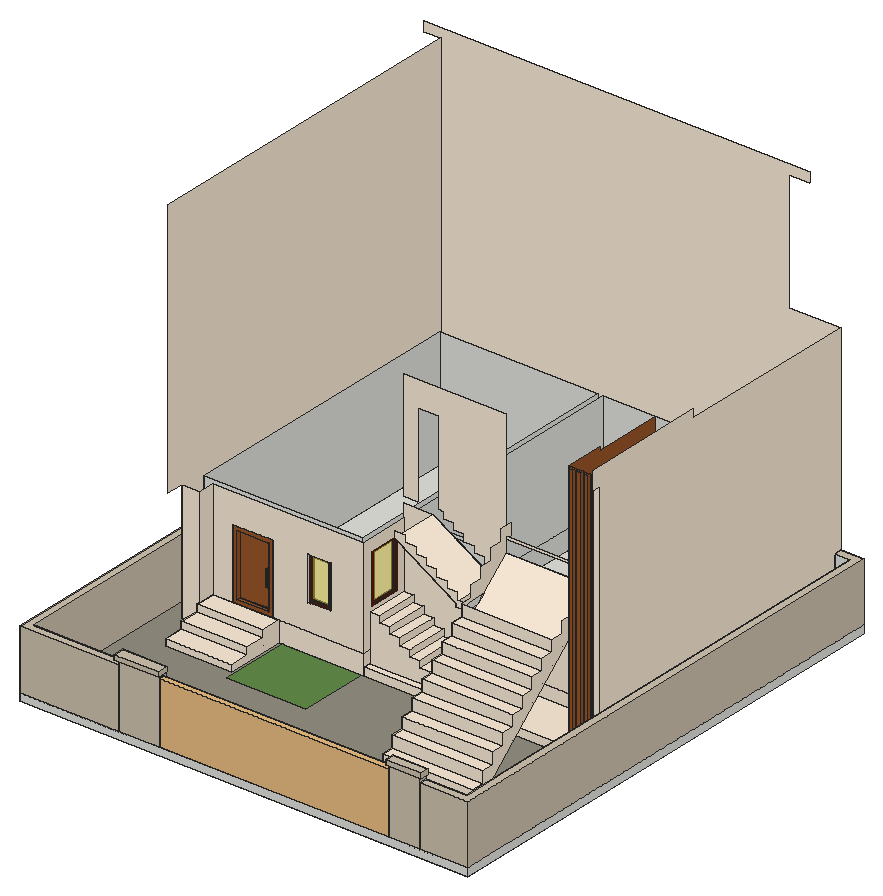
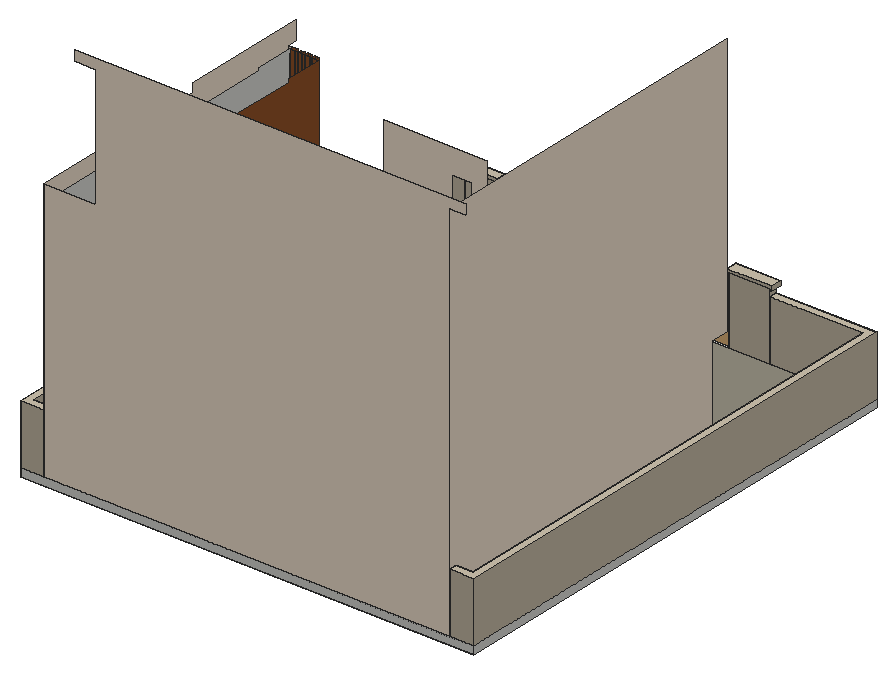
# SketchUp Ruby script. Lengths in inches.
U = 1.inch
M = Sketchup.active_model
def pt(a) = Geom::Point3d.new(a.map { |v| v * U })
def face(e, loops, mat)
  f = e.add_face(loops[0].map { |a| pt(a) })
  loops[1..].each { |l| e.add_face(l.map { |a| pt(a) }).erase! }
  f.material = f.back_material = mat if mat
  f
end
# faces: each face lists its corners as indices into pts; further lists are holes
def faces(e, pts, list, mat = nil) = list.each { |f| face(e, (f[0].is_a?(Array) ? f : [f]).map { |l| l.map { |i| pts[i] } }, mat) }
# xy, xz, yz: faces in a plane at the given z, y or x. An outline is a flat list of corners, or four numbers for a rectangle; further outlines are holes
def ring(l) = l.size == 4 ? [[l[0], l[1]], [l[2], l[1]], [l[2], l[3]], [l[0], l[3]]] : l.each_slice(2).to_a
def flat(e, list, mat, &to3) = list.each { |f| face(e, (f[0].is_a?(Array) ? f : [f]).map { |l| ring(l).map { |u, v| to3.(u, v) } }, mat) }
def xy(e, z, list, mat = nil) = flat(e, list, mat) { |x, y| [x, y, z] }
def xz(e, y, list, mat = nil) = flat(e, list, mat) { |x, z| [x, y, z] }
def yz(e, x, list, mat = nil) = flat(e, list, mat) { |y, z| [x, y, z] }
def lines(e, pts, list) = list.each { |a, b| e.add_line(pt(pts[a]), pt(pts[b])) }
# prism: a flat outline (further loops are holes) pulled along v
def prism(e, loops, v, mat = nil)
  f = face(e, loops, mat); d = Geom::Vector3d.new(v.map { |x| x * U })
  f.pushpull(f.normal.samedirection?(d) ? d.length : -d.length)
end
def box(e, o, s, mat = nil) = prism(e, [[o, [o[0] + s[0], o[1], o[2]], [o[0] + s[0], o[1] + s[1], o[2]], [o[0], o[1] + s[1], o[2]]]], [0, 0, s[2]], mat)
def at(x, y, z, deg = 0) = Geom::Transformation.translation(pt([x, y, z])) * Geom::Transformation.rotation(ORIGIN, Z_AXIS, deg.degrees)
def axes(o, x, y, z) = Geom::Transformation.new([*x, 0, *y, 0, *z, 0, *pt(o).to_a, 1])
def part(name) = M.definitions.add(name)
# library, detail: a bought-in or finely detailed component or shape, given as its bounding box
def library(name, o, s) = part(name).tap { |d| box(d.entities, o, s) }
def detail(e, o, s) = box(e.add_group.entities, o, s)
def put(e, d, t, mat = nil) = e.add_instance(d, t).tap { |i| i.material = mat if mat }
def group(e, t, mat = nil) = e.add_group.tap { |g| g.transformation = t; g.material = mat if mat }.entities
root = M.entities
M.materials.add("[0028_AntiqueWhite]").color = [250, 235, 215]
M.materials.add("[Color B08]").color = [102, 25, 0]
M.materials.add("[Metal Seamed]").color = [118, 119, 115]
M.materials.add("[Pavers Modular Brick]").color = [147, 143, 129]
M.materials.add("[Siding Rusty Metal]").color = [206, 195, 174]
M.materials.add("[Translucent Glass Blue]").color = [255, 231, 67]
M.materials["[Translucent Glass Blue]"].alpha = 0.5
M.materials.add("[Vegetation Grass Artificial]").color = [98, 140, 74]
M.materials.add("[Wood Board Cork]").color = [215, 201, 115]
M.materials.add("[Wood Cherry Original]").color = [152, 86, 42]
c1 = library("gate 512k",[0,0,0],[179,6.5,74.5])
c2 = part("Group\#3")
xy(c2.entities,0,[[0,0,22,2.875],[0,2.875,22,5.5]],"[Color B08]")
xy(c2.entities,2.22,[[2.22,0,19.78,2.875],[2.22,2.875,19.78,5.5]],"[Color B08]")
xy(c2.entities,55.28,[[2.22,0,19.78,2.875],[2.22,2.875,19.78,5.5]],"[Color B08]")
xy(c2.entities,57.5,[[0,0,22,2.875],[0,2.875,22,5.5]],"[Color B08]")
xz(c2.entities,0,[[[0,0,22,57.5],[2.22,2.22,19.78,55.28]]],"[Color B08]")
xz(c2.entities,2.875,[[[0,0,22,57.5],[2.22,2.22,19.78,55.28]]],"[Color B08]")
xz(c2.entities,2.875,[[2.22,2.22,19.78,55.28]],"[Translucent Glass Blue]")
xz(c2.entities,5.5,[[[0,0,22,57.5],[2.22,2.22,19.78,55.28]]],"[Color B08]")
yz(c2.entities,0,[[0,0,2.875,57.5],[2.875,0,5.5,57.5]],"[Color B08]")
yz(c2.entities,2.22,[[0,2.22,2.875,55.28],[2.875,2.22,5.5,55.28]],"[Color B08]")
yz(c2.entities,19.78,[[0,2.22,2.875,55.28],[2.875,2.22,5.5,55.28]],"[Color B08]")
yz(c2.entities,22,[[0,0,2.875,57.5],[2.875,0,5.5,57.5]],"[Color B08]")
xy(root,0,[[0,4.125,540,601.9375]])
xy(root,9,[[0,4.125,0,601.9375,29.1875,601.9375,29.1875,592.9375,9,592.9375,9,13.125,119.55,13.125,119.55,4.125],[119.55,4.125,168.34,13.125],[168.34,4.125,445.51,13.125],[445.51,4.125,482.875,13.125],[482.875,4.125,482.875,13.125,532.125,13.125,531,70.9375,531,592.9375,512.4375,592.9375,512.4375,601.9375,540,601.9375,540,4.125],
  [355.75,106.24,465.14,121.14],[50.75,159.9375,130.47,183.9375],[50.75,183.9375,130.47,212.0625],[[29.1875,212.0625,29.1875,601.9375,512.4375,601.9375,512.4375,292.4375,232.3125,292.4375,232.3125,231.9375,50.75,231.9375,50.75,212.0625],[232.3125,298.4375,506.4375,592.9375],[35.1875,237.9375,226.3125,592.9375]],[50.75,212.0625,130.47,231.9375],
  [232.3125,231.9375,512.4375,292.4375],[35.1875,237.9375,226.3125,592.9375],[232.3125,298.4375,506.4375,592.9375]])
xy(root,9,[[[9,13.125,532.125,13.125,531,70.9375,531,592.9375,512.4375,592.9375,512.4375,231.9375,230.49,231.9375,230.49,147.4375,134.99,147.4375,134.99,231.9375,130.47,231.9375,130.47,159.9375,50.75,159.9375,50.75,212.0625,29.1875,212.0625,29.1875,592.9375,9,592.9375],[355.75,106.24,465.14,121.14]]],"[Pavers Modular Brick]")
xy(root,9,[[134.99,147.4375,230.49,231.9375]],"[Vegetation Grass Artificial]")
xy(root,17,[[50.75,159.9375,130.47,183.9375]],"[0028_AntiqueWhite]")
xy(root,18,[[232.3125,231.9375,512.4375,231.9375,512.4375,238.0625,503.75,238.0625,503.75,242.8125,497.73,242.8125,497.73,246.875,494.11,246.875,494.11,242.8125,489.36,242.8125,489.36,246.875,485.67,246.875,485.67,242.8125,480.23,242.8125,480.23,246.875,476.92,246.875,476.92,242.8125,471.79,242.8125,471.79,246.875,468.75,246.875,468.75,292.4375,232.3125,292.4375]],"[0028_AntiqueWhite]")
xy(root,18,[[471.79,242.8125,476.92,246.875],[480.23,242.8125,485.67,246.875],[489.36,242.8125,494.11,246.875],[497.73,242.8125,503.75,246.875]],"[Wood Cherry Original]")
xy(root,22.73,[[355.75,106.24,465.14,121.14]],"[0028_AntiqueWhite]")
xy(root,25,[[50.75,183.9375,130.47,207.9375]],"[0028_AntiqueWhite]")
xy(root,33,[[74.72,231.9375,122.72,237.9375]])
xy(root,33,[[50.75,207.9375,130.47,231.9375]],"[0028_AntiqueWhite]")
xy(root,36.46,[[355.75,121.14,465.14,136.04]],"[0028_AntiqueWhite]")
xy(root,50.19,[[355.75,136.04,465.14,150.93]],"[0028_AntiqueWhite]")
xy(root,63.92,[[355.75,150.93,465.14,165.83]],"[0028_AntiqueWhite]")
xy(root,64.67,[[165.3125,231.9375,192.5,237.9375]])
xy(root,77.39,[[226.3125,243.1,232.3125,283.98]],"[0028_AntiqueWhite]")
xy(root,77.65,[[355.75,165.83,465.14,180.72]],"[0028_AntiqueWhite]")
xy(root,81,[[0,4.125,119.55,4.125,119.55,13.125,9,13.125,9,592.9375,29.1875,592.9375,29.1875,601.9375,0,601.9375],[482.875,4.125,540,4.125,540,601.9375,512.4375,601.9375,512.4375,592.9375,531,592.9375,531,70.9375,532.125,13.125,482.875,13.125]],"[Siding Rusty Metal]")
xy(root,86.9375,[[482.875,4.125,484.875,13.125]])
xy(root,86.9375,[[443.01,2.1875,484.875,4.125],[443.01,4.125,445.51,13.125]],"[Siding Rusty Metal]")
xy(root,87.4375,[[116.98,0,119.55,13.125],[119.55,0,170.53,4.125],[168.34,4.125,170.53,13.125]])
xy(root,88.6875,[[119.55,4.125,168.34,13.125],[445.51,4.125,482.875,13.125]])
xy(root,91.38,[[355.75,180.72,465.14,195.62]],"[0028_AntiqueWhite]")
xy(root,93,[[116.98,0,170.53,13.125],[443.01,2.1875,484.875,13.125]],"[Siding Rusty Metal]")
xy(root,105.11,[[355.75,195.62,465.14,210.51]],"[0028_AntiqueWhite]")
xy(root,117,[[74.72,231.9375,122.72,237.9375]])
xy(root,117.23,[[165.3125,231.9375,192.5,237.9375]])
xy(root,118.84,[[355.75,210.51,465.14,225.41]],"[0028_AntiqueWhite]")
xy(root,121,[[341.16,234.5,343.21,292.4375],[343.21,234.5,355.75,292.4375]],"[0028_AntiqueWhite]")
xz(root,0,[[116.98,87.4375,170.53,93]],"[Siding Rusty Metal]")
xz(root,2.1875,[[443.01,86.9375,484.875,93]],"[Siding Rusty Metal]")
xz(root,4.125,[[0,0,540,9],[445.51,86.9375,482.875,88.6875],[119.55,87.4375,168.34,88.6875]])
xz(root,4.125,[[0,9,119.55,81],[119.55,9,168.34,87.4375],[445.51,9,482.875,86.9375],[482.875,9,540,81]],"[Siding Rusty Metal]")
xz(root,13.125,[[9,9,119.55,81],[119.55,9,168.34,88.6875],[445.51,9,482.875,88.6875],[482.875,9,532.125,81],[443.01,86.9375,443.01,93,484.875,93,484.875,86.9375,482.875,86.9375,482.875,88.6875,445.51,88.6875,445.51,86.9375],
  [116.98,87.4375,116.98,93,170.53,93,170.53,87.4375,168.34,87.4375,168.34,88.6875,119.55,88.6875,119.55,87.4375]],"[Siding Rusty Metal]")
xz(root,106.24,[[355.75,9,465.14,22.73]],"[0028_AntiqueWhite]")
xz(root,121.14,[[355.75,22.73,465.14,36.46]],"[0028_AntiqueWhite]")
xz(root,136.04,[[355.75,36.46,465.14,50.19]],"[0028_AntiqueWhite]")
xz(root,150.93,[[355.75,50.19,465.14,63.92]],"[0028_AntiqueWhite]")
xz(root,159.9375,[[50.75,9,130.47,17]],"[0028_AntiqueWhite]")
xz(root,165.83,[[355.75,63.92,465.14,77.65]],"[0028_AntiqueWhite]")
xz(root,180.72,[[355.75,77.65,465.14,91.38]],"[0028_AntiqueWhite]")
xz(root,183.9375,[[50.75,17,130.47,25]],"[0028_AntiqueWhite]")
xz(root,195.62,[[355.75,91.38,465.14,105.11]],"[0028_AntiqueWhite]")
xz(root,207.9375,[[50.75,25,130.47,33]],"[0028_AntiqueWhite]")
xz(root,210.51,[[355.75,105.11,465.14,118.84]],"[0028_AntiqueWhite]")
xz(root,212.0625,[[29.1875,9,50.75,153]],"[0028_AntiqueWhite]")
xz(root,225.41,[[355.75,118.84,465.14,132.57]],"[0028_AntiqueWhite]")
xz(root,231.9375,[[50.75,9,130.47,25],[50.75,25,130.47,33]])
xz(root,231.9375,[[130.47,9,232.3125,33],[232.3125,9,512.4375,18],[[50.75,33,74.72,33,74.72,117,122.72,117,122.72,33,232.3125,33,232.3125,153,50.75,153],[165.3125,64.67,192.5,117.23]]],"[0028_AntiqueWhite]")
xz(root,234.5,[[341.16,121,355.75,121,355.75,129,343.21,129,343.21,137,330.68,137,330.68,145,318.14,145,318.14,153,305.61,153,305.61,161,293.07,161,293.07,169,280.54,169,280.54,177,268,177,268,169,341.16,124.92]],"[0028_AntiqueWhite]")
xz(root,237.9375,[[35.1875,9,226.3125,33],[[35.1875,33,35.1875,153,226.3125,153,226.3125,33,122.72,33,122.72,117,74.72,117,74.72,33],[165.3125,64.67,192.5,117.23]]])
xz(root,238.0625,[[503.75,18,512.4375,309]],"[0028_AntiqueWhite]")
xz(root,242.8125,[[471.79,18,476.92,312.375],[480.23,18,485.67,312.375],[489.36,18,494.11,312.375],[497.73,18,503.75,312.375]],"[Wood Cherry Original]")
xz(root,243.1,[[226.3125,77.39,232.3125,138.45]])
xz(root,246.875,[[468.75,18,471.79,312.375],[471.79,18,476.92,312.375],[476.92,18,480.23,312.375],[480.23,18,485.67,312.375],[485.67,18,489.36,312.375],
  [489.36,18,494.11,312.375],[494.11,18,497.73,312.375],[497.73,18,503.75,312.375]],"[Wood Cherry Original]")
xz(root,283.98,[[226.3125,77.39,232.3125,138.45]],"[0028_AntiqueWhite]")
xz(root,292.4375,[[232.3125,9,355.625,18],[468.75,18,503.75,177],[341.16,121,341.16,124.92,294.56,153,318.14,153,318.14,145,330.68,145,330.68,137,343.21,137,343.21,129,355.75,129,355.75,121]])
xz(root,292.4375,[[232.3125,18,468.75,33],[232.3125,33,468.75,33,468.75,177,355.625,177,355.75,173.76,465.14,173.76,465.14,159.01,355.75,159.01,355.75,173.76,355.625,177,355.625,309,232.3125,309,232.3125,177,249.93,177,249.93,278.54,274.3,278.54,274.3,177,280.54,177,280.54,169,293.07,169,293.07,161,305.61,161,305.61,153,318.14,153,318.14,145,330.68,145,330.68,137,343.21,137,343.21,129,355.75,129,355.75,121,341.16,121,341.16,124.92,294.56,153,268,169,232.3125,169]],"[0028_AntiqueWhite]")
xz(root,298.4375,[[232.3125,9,506.4375,33],[232.3125,33,506.4375,153]])
xz(root,592.9375,[[9,9,29.1875,81],[35.1875,9,226.3125,33],[232.3125,9,506.4375,33],[512.4375,9,531,81],[35.1875,33,226.3125,153],
  [232.3125,33,506.4375,153]])
xz(root,601.9375,[[0,0,540,9]])
xz(root,601.9375,[[29.1875,9,29.1875,465,9.6875,465,9.6875,477,475.6875,477,475.6875,465,450.25,465,450.25,321,512.4375,321,512.4375,9]],"[0028_AntiqueWhite]")
xz(root,601.9375,[[0,9,29.1875,81],[512.4375,9,540,81]],"[Siding Rusty Metal]")
yz(root,0,[[4.125,0,601.9375,9]])
yz(root,0,[[4.125,9,601.9375,81]],"[Siding Rusty Metal]")
yz(root,9,[[13.125,9,592.9375,81]],"[Siding Rusty Metal]")
yz(root,29.1875,[[592.9375,9,601.9375,81]])
yz(root,29.1875,[[212.0625,9,212.0625,153,190.5,153,190.5,465,601.9375,465,601.9375,81,592.9375,81,592.9375,9]],"[0028_AntiqueWhite]")
yz(root,35.1875,[[237.9375,9,592.9375,153]])
yz(root,50.75,[[212.0625,9,231.9375,25],[212.0625,25,231.9375,33]])
yz(root,50.75,[[159.9375,9,159.9375,17,183.9375,17,183.9375,25,207.9375,25,207.9375,33,212.0625,33,212.0625,9],[212.0625,33,231.9375,153]],"[0028_AntiqueWhite]")
yz(root,74.72,[[231.9375,33,237.9375,117]])
yz(root,116.98,[[0,87.4375,13.125,93]],"[Siding Rusty Metal]")
yz(root,119.55,[[4.125,9,13.125,81],[4.125,87.4375,13.125,88.6875]])
yz(root,119.55,[[4.125,81,13.125,87.4375]],"[Siding Rusty Metal]")
yz(root,122.72,[[231.9375,33,237.9375,117]])
yz(root,130.47,[[159.9375,9,231.9375,9,231.9375,33,207.9375,33,207.9375,25,183.9375,25,183.9375,17,159.9375,17]],"[0028_AntiqueWhite]")
yz(root,165.3125,[[231.9375,64.67,237.9375,117.23]])
yz(root,168.34,[[4.125,87.4375,13.125,88.6875]])
yz(root,168.34,[[4.125,9,13.125,87.4375]],"[Siding Rusty Metal]")
yz(root,170.53,[[0,87.4375,13.125,93]],"[Siding Rusty Metal]")
yz(root,192.5,[[231.9375,64.67,237.9375,117.23]])
yz(root,226.3125,[[237.9375,9,592.9375,33],[[237.9375,33,592.9375,153],[243.1,77.39,283.98,138.45]]])
yz(root,232.3125,[[231.9375,9,292.4375,18],[298.4375,9,592.9375,33],[298.4375,33,592.9375,153]])
yz(root,232.3125,[[231.9375,18,292.4375,33],[[231.9375,33,292.4375,153],[243.1,77.39,283.98,138.45]]],"[0028_AntiqueWhite]")
yz(root,341.16,[[234.5,121,292.4375,124.92]],"[0028_AntiqueWhite]")
yz(root,355.75,[[234.5,121,234.5,129,258.17,129,249.03,121]])
yz(root,355.75,[[106.24,9,106.24,22.73,121.14,22.73,121.14,36.46,136.04,36.46,136.04,50.19,150.93,50.19,150.93,63.92,165.83,63.92,165.83,77.65,180.72,77.65,180.72,91.38,195.62,91.38,195.62,105.11,210.51,105.11,210.51,118.84,225.41,118.84,225.41,132.57,240.3,132.57,240.3,146.3,255.2,146.3,255.2,160.03,270.09,160.03,270.09,173.76,284.99,173.76,284.99,187.49,299.89,187.49,299.89,173.76,292.4375,173.76,292.4375,159.01,258.17,129,234.5,129,234.5,121,249.03,121,121.14,9],[249.03,121,292.4375,121,292.4375,129,258.17,129]],"[0028_AntiqueWhite]")
yz(root,443.01,[[2.1875,86.9375,13.125,93]],"[Siding Rusty Metal]")
yz(root,445.51,[[4.125,86.9375,13.125,88.6875]])
yz(root,445.51,[[4.125,9,13.125,86.9375]],"[Siding Rusty Metal]")
yz(root,465.14,[[106.24,9,121.14,9,292.4375,159.01,292.4375,173.76,284.99,173.76,284.99,160.03,270.09,160.03,270.09,146.3,240.3,146.3,240.3,132.57,225.41,132.57,225.41,118.84,210.51,118.84,210.51,105.11,195.62,105.11,195.62,91.38,180.72,91.38,180.72,77.65,165.83,77.65,165.83,63.92,150.93,63.92,150.93,50.19,136.04,50.19,136.04,36.46,121.14,36.46,121.14,22.73,106.24,22.73]],"[0028_AntiqueWhite]")
yz(root,468.75,[[246.875,18,246.875,312.375,292.4375,312.375,292.4375,309,376.0625,309,376.0625,177,292.4375,177,292.4375,18]],"[Wood Cherry Original]")
yz(root,471.79,[[242.8125,18,246.875,312.375]],"[Wood Cherry Original]")
yz(root,476.92,[[242.8125,18,246.875,312.375]],"[Wood Cherry Original]")
yz(root,480.23,[[242.8125,18,246.875,312.375]],"[Wood Cherry Original]")
yz(root,482.875,[[4.125,9,13.125,81],[4.125,86.9375,13.125,88.6875]])
yz(root,482.875,[[4.125,81,13.125,86.9375]],"[Siding Rusty Metal]")
yz(root,484.875,[[2.1875,86.9375,13.125,93]],"[Siding Rusty Metal]")
yz(root,485.67,[[242.8125,18,246.875,312.375]],"[Wood Cherry Original]")
yz(root,489.36,[[242.8125,18,246.875,312.375]],"[Wood Cherry Original]")
yz(root,494.11,[[242.8125,18,246.875,312.375]],"[Wood Cherry Original]")
yz(root,497.73,[[242.8125,18,246.875,312.375]],"[Wood Cherry Original]")
yz(root,503.75,[[238.0625,18,242.8125,33],[246.875,18,292.4375,18,292.4375,177,592.9375,177,592.9375,309,292.4375,309,292.4375,312.375,246.875,312.375]])
yz(root,503.75,[[238.0625,33,242.8125,309]],"[0028_AntiqueWhite]")
yz(root,503.75,[[242.8125,18,246.875,33],[242.8125,33,246.875,309]],"[Wood Cherry Original]")
yz(root,506.4375,[[298.4375,9,592.9375,33],[298.4375,33,592.9375,153]])
yz(root,512.4375,[[592.9375,9,601.9375,81]])
yz(root,512.4375,[[231.9375,9,592.9375,9,592.9375,81,601.9375,81,601.9375,321,379.25,321,379.25,331.3125,227.125,331.3125,227.125,309,238.0625,309,238.0625,18,231.9375,18]],"[0028_AntiqueWhite]")
yz(root,531,[[70.9375,9,592.9375,81]],"[Siding Rusty Metal]")
yz(root,540,[[4.125,0,601.9375,9]])
yz(root,540,[[4.125,9,601.9375,81]],"[Siding Rusty Metal]")
p = [[531,70.9375,9],[532.125,13.125,9],[532.125,13.125,81],[531,70.9375,81],[355.75,258.17,129],[355.75,292.4375,159.01],
  [465.14,292.4375,159.01],[465.14,121.14,9],[355.75,121.14,9],[355.75,249.03,121],[341.16,234.5,124.92],[268,234.5,169],
  [268,292.4375,169],[294.56,292.4375,153],[341.16,292.4375,124.92],[503.75,292.4375,18],[512.4375,292.4375,18],[50.75,207.9375,17],
  [130.47,207.9375,17],[355.75,165.83,50.19],[465.14,165.83,50.19],[355.75,180.72,63.92],[465.14,180.72,63.92],[355.75,195.62,77.65],
  [465.14,195.62,77.65],[355.75,210.51,91.38],[465.14,210.51,91.38],[355.75,225.41,105.11],[465.14,225.41,105.11],[355.75,240.3,118.84],
  [465.14,240.3,118.84]]
faces(root,p,[[0,1,2,3]],"[Siding Rusty Metal]")
faces(root,p,[[4,5,6,7,8,9],[10,11,12,13,14]],"[0028_AntiqueWhite]")
lines(root,p,[[15,16],[17,18],[19,20],[21,22],[23,24],[25,26],[27,28],[29,30]])
put(root,c1,axes([445.51,4.125,9],[-1.54842,0,0],[0,1,0],[0,0,1]),"[Wood Board Cork]")
g1 = group(root,at(232.3125,241.32,18),"[0028_AntiqueWhite]")
prism(g1,[[[72,51.12,16],[72,51.12,8],[84,51.12,8],[84,51.12,0],[72,51.12,0],[0,51.12,0],[0,51.12,48],[0,51.12,56],[12,51.12,56],[12,51.12,48],[24,51.12,48],[24,51.12,40],[36,51.12,40],[36,51.12,32],[48,51.12,32],[48,51.12,24],[60,51.12,24],[60,51.12,16]]],[0,-51.12,0])
g2 = group(root,at(74.72,231.9375,33))
xy(g2,0,[[0,0,48,4.9375]],"[Wood Cherry Original]")
xy(g2,4.41,[[4.41,0,43.59,4.9375]],"[Wood Cherry Original]")
xy(g2,29.35,[[37.76,1.9375,40.2,4.9375]],"[Metal Seamed]")
xy(g2,48.73,[[37.76,1.9375,40.2,4.9375]],"[Metal Seamed]")
xy(g2,79.59,[[4.41,0,43.59,4.9375]],"[Wood Cherry Original]")
xy(g2,84,[[0,0,48,4.9375]],"[Wood Cherry Original]")
xz(g2,0,[[[0,0,48,84],[4.41,4.41,43.59,79.59]]],"[Wood Cherry Original]")
xz(g2,1.9375,[[37.76,29.35,40.2,48.73]],"[Metal Seamed]")
xz(g2,4.9375,[[37.76,29.35,40.2,48.73]],"[Metal Seamed]")
xz(g2,4.9375,[[[0,0,48,84],[4.41,4.41,43.59,79.59]],[[4.41,4.41,43.59,79.59],[37.76,29.35,40.2,48.73]]],"[Wood Cherry Original]")
yz(g2,0,[[0,0,4.9375,84]],"[Wood Cherry Original]")
yz(g2,4.41,[[0,4.41,4.9375,79.59]],"[Wood Cherry Original]")
yz(g2,37.76,[[1.9375,29.35,4.9375,48.73]],"[Metal Seamed]")
yz(g2,40.2,[[1.9375,29.35,4.9375,48.73]],"[Metal Seamed]")
yz(g2,43.59,[[0,4.41,4.9375,79.59]],"[Wood Cherry Original]")
yz(g2,48,[[0,0,4.9375,84]],"[Wood Cherry Original]")
put(root,c2,axes([165.3125,232.76,64.67],[1.2358,0,0],[0,0.85,0],[0,0,0.91413]))
put(root,c2,axes([232.3125,243.1,77.39],[0,1.85795,0],[-0.85,0,0],[0,0,1.06196]))
